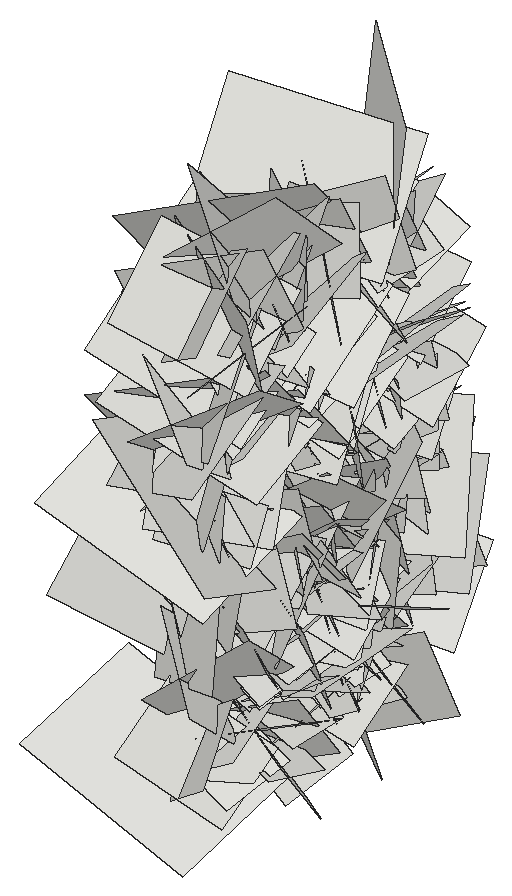
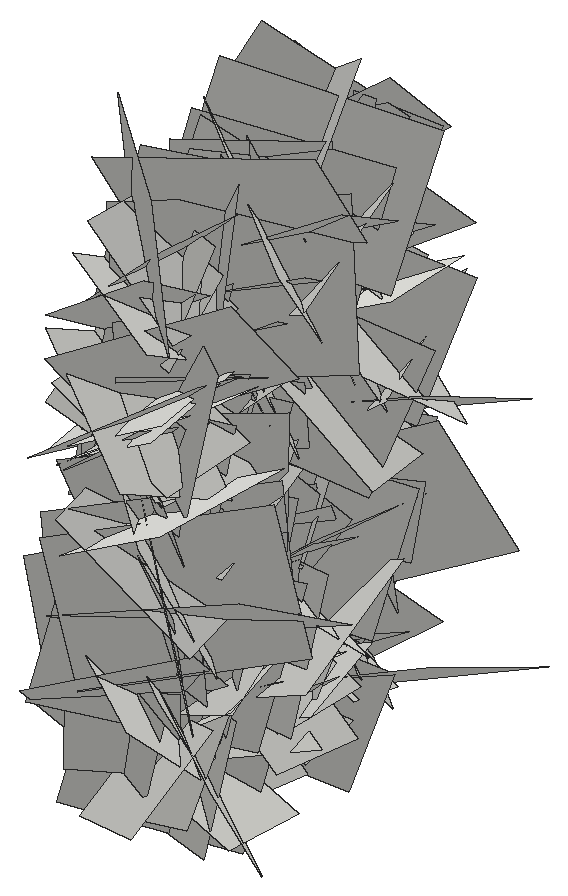
# SketchUp Ruby script. Lengths in inches.
U = 1.inch
M = Sketchup.active_model
def pt(a) = Geom::Point3d.new(a.map { |v| v * U })
def face(e, loops, mat)
  f = e.add_face(loops[0].map { |a| pt(a) })
  loops[1..].each { |l| e.add_face(l.map { |a| pt(a) }).erase! }
  f.material = f.back_material = mat if mat
  f
end
# faces: each face lists its corners as indices into pts; further lists are holes
def faces(e, pts, list, mat = nil) = list.each { |f| face(e, (f[0].is_a?(Array) ? f : [f]).map { |l| l.map { |i| pts[i] } }, mat) }
# xy, xz, yz: faces in a plane at the given z, y or x. An outline is a flat list of corners, or four numbers for a rectangle; further outlines are holes
def ring(l) = l.size == 4 ? [[l[0], l[1]], [l[2], l[1]], [l[2], l[3]], [l[0], l[3]]] : l.each_slice(2).to_a
def flat(e, list, mat, &to3) = list.each { |f| face(e, (f[0].is_a?(Array) ? f : [f]).map { |l| ring(l).map { |u, v| to3.(u, v) } }, mat) }
def xy(e, z, list, mat = nil) = flat(e, list, mat) { |x, y| [x, y, z] }
def xz(e, y, list, mat = nil) = flat(e, list, mat) { |x, z| [x, y, z] }
def yz(e, x, list, mat = nil) = flat(e, list, mat) { |y, z| [x, y, z] }
def lines(e, pts, list) = list.each { |a, b| e.add_line(pt(pts[a]), pt(pts[b])) }
# prism: a flat outline (further loops are holes) pulled along v
def prism(e, loops, v, mat = nil)
  f = face(e, loops, mat); d = Geom::Vector3d.new(v.map { |x| x * U })
  f.pushpull(f.normal.samedirection?(d) ? d.length : -d.length)
end
def box(e, o, s, mat = nil) = prism(e, [[o, [o[0] + s[0], o[1], o[2]], [o[0] + s[0], o[1] + s[1], o[2]], [o[0], o[1] + s[1], o[2]]]], [0, 0, s[2]], mat)
def at(x, y, z, deg = 0) = Geom::Transformation.translation(pt([x, y, z])) * Geom::Transformation.rotation(ORIGIN, Z_AXIS, deg.degrees)
def axes(o, x, y, z) = Geom::Transformation.new([*x, 0, *y, 0, *z, 0, *pt(o).to_a, 1])
def part(name) = M.definitions.add(name)
# library, detail: a bought-in or finely detailed component or shape, given as its bounding box
def library(name, o, s) = part(name).tap { |d| box(d.entities, o, s) }
def detail(e, o, s) = box(e.add_group.entities, o, s)
def put(e, d, t, mat = nil) = e.add_instance(d, t).tap { |i| i.material = mat if mat }
def group(e, t, mat = nil) = e.add_group.tap { |g| g.transformation = t; g.material = mat if mat }.entities
root = M.entities
c1 = part("Component\#6")
p = [[0.01,0,0],[0,3.24,4.54],[4.32,3.24,4.54],[4.33,0,0]]
faces(c1.entities,p,[[0,1,2,3]])
put(root,c1,axes([404.88,161.87,9.58],[-0.35888,-0.49511,-1.17449],[-0.11741,-1.19919,0.53746],[-1.34594,0.23663,0.26628]))
put(root,c1,axes([404.88,170.67,8.29],[-0.13658,-1.14766,-0.62909],[-0.33753,-0.58565,1.13362],[-1.34561,0.26339,-0.2205]))
put(root,c1,axes([404.88,160.65,1.35],[-0.1594,-1.22011,-0.46707],[-0.28659,-0.43091,1.2127],[-1.35486,0.2347,-0.20157]))
put(root,c1,axes([404.88,161.24,11.55],[-0.08722,-1.18104,-0.51149],[-0.30261,-0.48302,1.16122],[-1.33028,0.18731,-0.23062]))
put(root,c1,axes([404.88,161.91,24.73],[-0.20116,0.87735,-0.9177],[-0.06395,-0.93308,-0.87958],[-1.34427,-0.0869,0.17917]))
put(root,c1,axes([404.88,167.61,21.95],[-0.32344,0.31012,-1.26322],[0.1451,-1.28265,-0.34796],[-1.37111,-0.2089,0.26116]))
put(root,c1,axes([404.88,171.01,11.29],[-0.23144,-0.15428,-1.27652],[0.01824,-1.29503,0.15357],[-1.36284,0.00887,0.21884]))
put(root,c1,axes([404.88,161.07,7.88],[-0.0926,0.91308,0.78861],[-0.24837,0.76278,-0.90913],[-1.25453,-0.21841,0.12178]))
put(root,c1,axes([404.88,170.58,10.37],[-0.24309,-1.14649,0.14454],[-0.04952,0.15643,1.16674],[-1.2239,0.22139,-0.07591]))
put(root,c1,axes([404.88,165.1,2.71],[0.06092,-1.21711,0.58199],[-0.18306,0.57109,1.21136],[-1.41828,-0.12599,-0.13136]))
put(root,c1,axes([404.88,162.31,11.53],[-0.17206,0.75955,-0.87532],[-0.12131,-0.89005,-0.75111],[-1.22246,-0.01858,0.19774]))
put(root,c1,axes([404.88,157.93,15.34],[-0.27083,1.19165,0.15594],[0.0802,0.17506,-1.21378],[-1.27139,-0.2428,-0.10978]))
put(root,c1,axes([404.88,168.375,23.9],[0.0952,-0.72561,-1.04974],[-0.29336,-1.03837,0.69407],[-1.32049,0.17837,-0.22987]))
put(root,c1,axes([404.88,159.14,18.38],[-0.07521,0.79304,-0.86536],[-0.12573,-0.86735,-0.78513],[-1.23784,0.03991,0.13233]))
put(root,c1,axes([404.88,155.03,14.95],[0.10989,1.07322,0.82249],[-0.07177,0.82799,-1.07186],[-1.43147,0.04087,0.11688]))
put(root,c1,axes([404.88,166.4,18.65],[0.092,-1.19571,-0.63762],[-0.0325,-0.6405,1.19693],[-1.43603,-0.06211,-0.06794]))
put(root,c1,axes([404.88,159.69,18.96],[-0.02704,0.74145,1.09535],[0.09362,1.09406,-0.73853],[-1.39894,0.05888,-0.07059]))
put(root,c1,axes([404.88,163.36,23.49],[-0.04873,0.57368,-1.00395],[-0.12423,-1.00188,-0.56714],[-1.21936,0.07915,0.09791]))
put(root,c1,axes([404.88,162.85,15.75],[-0.04254,-1.00522,0.67204],[-0.02385,0.67292,1.00519],[-1.28151,0.02084,-0.04102]))
put(root,c1,axes([404.88,163.86,1.73],[-0.03729,0.66749,1.03354],[0.00972,1.03407,-0.66752],[-1.30413,-0.01138,-0.03452]))
put(root,c1,axes([404.88,161.03,16.77],[0.02327,0.73455,-0.90907],[-0.17416,-0.89826,-0.72978],[-1.22657,0.14148,0.08637]))
put(root,c1,axes([404.88,162.03,18.62],[-0.15865,-0.78055,-0.79386],[0.03617,-0.80384,0.78393],[-1.17956,0.08034,0.13081]))
put(root,c1,axes([404.88,161.02,12.77],[-0.04866,0.36936,-1.04237],[-0.12613,-1.03886,-0.36288],[-1.16543,0.09701,0.0828]))
put(root,c1,axes([404.88,163.21,2.24],[0.08398,-0.53221,1.10764],[-0.11648,1.10243,0.53756],[-1.29738,-0.13342,0.02343]))
put(root,c1,axes([404.88,155.93,16.01],[-0.06166,0.77521,1.08886],[0.24821,1.07895,-0.75564],[-1.39492,0.15772,-0.18259]))
put(root,c1,axes([400.91,164.09,3.1],[-0.16189,-0.51758,0.36968],[-0.06161,0.38995,0.52196],[0.67139,-0.08902,0.13704]))
put(root,c1,axes([404.88,165.97,13.03],[-0.11695,-0.23373,1.15092],[0.10796,1.14973,0.24325],[-1.24018,0.12213,-0.08736]))
put(root,c1,axes([404.88,170.79,17.67],[-0.07972,-0.69903,-0.88266],[0.01234,-0.88506,0.69994],[-1.19343,0.03754,0.0662]))
put(root,c1,axes([404.88,164.53,2.65],[-0.11418,0.95876,0.15487],[-0.16789,0.13639,-0.95453],[-1.01568,-0.13033,0.14037]))
put(root,c1,axes([404.88,165.6875,8.33],[-0.14254,-0.77018,0.64298],[-0.05856,0.65343,0.77114],[-1.06187,0.06735,-0.12884]))
put(root,c1,axes([400.91,159.77,13.93],[-0.14822,0.47929,0.38572],[0.01533,0.39801,-0.48932],[0.65196,0.0996,0.0992]))
put(root,c1,axes([404.88,164.18,5.53],[-0.00871,-1.21515,-0.1589],[0.11926,-0.15898,1.20995],[-1.29354,-0.00648,0.11262]))
put(root,c1,axes([404.88,168.99,0.33],[-0.20008,-0.71049,0.66963],[0.07161,0.67089,0.73087],[-1.03242,0.18422,-0.07908]))
put(root,c1,axes([404.88,166.625,12.7],[-0.17127,1.04033,-0.10676],[0.13463,-0.08771,-1.04688],[-1.10034,-0.17266,-0.11147]))
put(root,c1,axes([404.88,160.14,4.78],[-0.03826,-0.47304,0.81506],[-0.18962,0.80427,0.45886],[-0.98077,-0.13704,-0.12051]))
put(root,c1,axes([400.91,170.02,6.34],[-0.13634,-0.30577,-0.6303],[-0.02329,-0.63876,0.31436],[0.74222,-0.07621,-0.10592]))
put(root,c1,axes([404.88,156.14,6.5],[-0.17845,0.35117,0.84391],[-0.01887,0.85668,-0.36003],[-0.96872,-0.08137,-0.14844]))
put(root,c1,axes([404.88,163.93,5.47],[-0.11462,-1.01834,-0.26907],[0.10191,-0.2789,1.0169],[-1.11183,0.07941,0.12095]))
put(root,c1,axes([400.91,162.91,7.6875],[-0.03517,0.6334,0.29771],[-0.1292,0.28826,-0.62688],[0.73053,0.08147,-0.09654]))
put(root,c1,axes([404.88,160.62,5.12],[-0.08568,1.04485,0.18773],[0.09569,0.19436,-1.04286],[-1.1212,-0.06325,-0.10335]))
put(root,c1,axes([404.88,162.44,14.8125],[0.22172,-1.13603,-0.19278],[-0.19013,-0.22565,1.13507],[-1.20652,-0.17321,-0.21429]))
put(root,c1,axes([404.88,159.91,9.22],[0.2022,-1.20502,0.50539],[0.1049,0.52261,1.20871],[-1.38114,-0.13672,0.1658]))
put(root,c1,axes([404.88,163.57,3.71],[-0.11292,-0.2033,0.99476],[0.09749,0.99417,0.21302],[-1.07181,0.11185,-0.08542]))
put(root,c1,axes([404.88,166.01,11.8],[-0.21466,0.53877,-0.68228],[0.03009,-0.69607,-0.55809],[-0.92102,-0.14831,0.14079]))
put(root,c1,axes([404.88,168.87,14.79],[-0.03205,0.06087,-1.12787],[0.16204,-1.11767,-0.06442],[-1.18627,-0.15431,0.02167]))
put(root,c1,axes([404.88,167.18,1.59],[0.07507,-1.0991,0.32301],[0.05871,0.32653,1.09895],[-1.2129,-0.05222,0.07319]))
put(root,c1,axes([404.88,157.18,19.73],[0.07599,0.81527,0.8297],[0.084,0.82592,-0.8184],[-1.23014,0.10676,-0.00463]))
put(root,c1,axes([404.88,167.28,17.92],[0.19972,-0.96368,-0.57877],[-0.14667,-0.60226,0.95775],[-1.18251,-0.08806,-0.21655]))
put(root,c1,axes([404.88,167.22,15.375],[0.0235,-0.92066,-0.53568],[0.01768,-0.53543,0.92093],[-1.12894,-0.02755,0.00327]))
put(root,c1,axes([400.91,162.79,15.86],[-0.07285,0.46729,0.4905],[0.02436,0.49435,-0.46773],[0.71769,0.03066,0.06566]))
put(root,c1,axes([400.91,161.25,17.66],[-0.25985,0.898,-0.37026],[-0.14737,-0.41038,-0.90325],[1.01902,0.16964,-0.22504]))
put(root,c1,axes([400.91,165.96,10.85],[-0.09912,0.20412,-0.70693],[-0.02587,-0.71308,-0.20267],[0.77953,0.00229,-0.09661]))
put(root,c1,axes([404.88,169.19,10.7],[0.0913,0.46499,-1.24639],[0.29576,-1.22753,-0.43867],[-1.37875,-0.23253,-0.17663]))
put(root,c1,axes([404.88,168.14,0.12],[0.06773,-0.63363,0.78179],[-0.11595,0.77435,0.63654],[-1.06038,-0.12515,-0.01967]))
put(root,c1,axes([404.88,166.18,19.56],[0.12535,0.0531,1.28965],[0.2192,1.27754,-0.07157],[-1.35051,0.21229,0.10808]))
put(root,c1,axes([404.88,167.01,8.33],[-0.18631,0.3359,0.73427],[-0.04897,0.74605,-0.35235],[-0.8545,-0.11599,-0.1399]))
put(root,c1,axes([400.91,159.82,10.86],[-0.164,0.05549,-0.7166],[0.119,-0.72215,-0.08015],[0.75252,0.12629,-0.14349]))
put(root,c1,axes([404.88,164.72,6.23],[0.02586,0.29335,1.1723],[0.23754,1.1511,-0.29271],[-1.25874,0.22326,-0.03115]))
put(root,c1,axes([400.91,164.71,11.17],[-0.09162,-0.23701,0.75882],[-0.09076,0.76162,0.22813],[0.83777,0.05659,0.1077]))
put(root,c1,axes([400.91,167.39,12.19],[-0.06725,0.11282,-0.6237],[0.12717,-0.61335,-0.12315],[0.65971,0.12973,-0.03984]))
put(root,c1,axes([400.91,158.25,7.85],[0.01053,0.60228,-0.51533],[-0.19634,-0.49934,-0.58716],[0.81696,-0.12777,-0.13447]))
put(root,c1,axes([404.88,165.51,17.74],[-0.00528,-0.97827,-0.44464],[0.11526,-0.44282,0.97306],[-1.13321,-0.04048,0.10104]))
put(root,c1,axes([404.88,165.75,-1.09],[0.03685,-0.4153,0.96157],[0.02645,0.96216,0.41465],[-1.10996,0.00914,0.04181]))
put(root,c1,axes([404.88,167.74,3.51],[0.11337,-0.86322,0.3774],[-0.28126,0.33685,0.84566],[-0.95821,-0.201,-0.20357]))
put(root,c1,axes([404.88,161.03,4.22],[-0.00206,0.54706,-0.73945],[-0.10036,-0.73565,-0.544],[-0.96983,0.07497,0.05787]))
put(root,c1,axes([404.88,158.84,13.7],[-0.15038,-0.75335,0.50607],[0.08727,0.49942,0.76653],[-0.95804,0.16374,-0.00961]))
put(root,c1,axes([404.88,166.72,20.27],[-0.14718,0.45385,-0.66356],[-0.05291,-0.67695,-0.45256],[-0.85051,-0.03642,0.14299]))
put(root,c1,axes([400.91,158.82,19.64],[0.09205,0.73549,-0.019],[-0.17536,0.00088,-0.72213],[0.75991,-0.08889,-0.16434]))
put(root,c1,axes([404.88,169.09,13.37],[-0.12805,-0.81492,0.2825],[0.01832,0.28292,0.8235],[-0.91406,0.11983,-0.02307]))
put(root,c1,axes([400.91,159.61,12.59],[0.0897,0.16152,-0.57424],[0.01993,-0.58042,-0.16049],[0.632,-0.00462,0.08656]))
put(root,c1,axes([400.91,160.65,18.69],[0.1336,-0.1743,0.59472],[-0.06624,0.60023,0.18916],[0.65357,0.09646,-0.1024]))
put(root,c1,axes([400.91,160.54,14.42],[-0.065,-0.29459,-0.75204],[-0.0763,-0.74921,0.29935],[0.85274,-0.0895,-0.03054]))
put(root,c1,axes([400.91,161.26,10.83],[-0.08958,0.45503,-0.59155],[0.06652,-0.58889,-0.46195],[0.78829,0.10141,-0.02824]))
put(root,c1,axes([404.88,170.16,13.55],[0.14984,-1.04824,-0.22204],[-0.00627,-0.22472,1.05715],[-1.13577,-0.13705,-0.03513]))
put(root,c1,axes([400.91,160.97,6.7],[0.04912,0.73058,0.10133],[-0.09877,0.10652,-0.72536],[0.77557,-0.03271,-0.0988]))
put(root,c1,axes([404.88,163.26,10.51],[-0.09772,0.8385,-0.3881],[0.10419,-0.37892,-0.842],[-0.97385,-0.12468,-0.05114]))
put(root,c1,axes([400.91,159.79,25.07],[-0.1328,0.69586,-0.68383],[-0.18687,-0.69425,-0.67416],[1.01714,-0.03669,-0.21313]))
put(root,c1,axes([404.88,167.39,3.05],[0.22625,-1.02118,-0.283],[-0.12014,-0.30902,1.02962],[-1.11681,-0.17363,-0.16809]))
put(root,c1,axes([400.91,159.32,12.84],[0.06752,-0.16321,-0.59207],[0.0871,-0.58763,0.17083],[0.64514,0.09641,0.0389]))
put(root,c1,axes([400.91,169.73,5.36],[0.07377,0.11031,-0.61615],[0.06228,-0.61836,-0.10407],[0.66058,0.04598,0.07863]))
put(root,c1,axes([404.88,166.22,16.78],[0.0558,0.90138,-0.08554],[-0.09664,-0.07998,-0.89882],[-0.95488,0.06076,0.08597]))
put(root,c1,axes([400.91,166.8,6.58],[-0.19077,-0.84984,-0.315],[0.00737,-0.32244,0.86593],[0.9607,-0.16629,-0.0692]))
put(root,c1,axes([404.88,159.03,23.29],[0.13252,0.38295,-0.87838],[-0.10893,-0.87536,-0.39626],[-1.00987,0.14467,-0.07253]))
put(root,c1,axes([400.91,160.57,3.12],[0.03509,0.82869,0.13415],[-0.15764,0.13792,-0.81528],[0.87577,-0.00838,-0.15213]))
put(root,c1,axes([400.91,164.04,15.7],[0.03624,-0.6234,-0.24842],[0.08,-0.24359,0.62167],[0.70683,0.05954,-0.05762]))
put(root,c1,axes([404.88,170.98,12.21],[0.31631,-0.51758,-1.19288],[0.16648,-1.20059,0.56021],[-1.36826,-0.26573,-0.20761]))
put(root,c1,axes([400.91,169.83,13.22],[0.13817,-0.64015,-0.16037],[-0.03989,-0.17041,0.64965],[0.69839,0.11692,0.06883]))
put(root,c1,axes([400.91,161.46,7.67],[0.11157,-0.00104,0.59962],[0.09459,0.60203,-0.01462],[0.62852,-0.09042,-0.10424]))
put(root,c1,axes([404.88,168.08,9.41],[0.11593,0.02752,-0.90523],[-0.14705,-0.90054,-0.04413],[-0.94866,0.14295,-0.10378]))
put(root,c1,axes([400.91,169.26,18.83],[0.02849,-0.83115,-0.05333],[-0.13283,-0.05679,0.82186],[0.87278,0.01849,0.12683]))
put(root,c1,axes([400.91,165.55,15.88],[-0.02597,-0.35934,-0.67832],[0.02345,-0.67872,0.35875],[0.81334,0.00809,-0.032]))
put(root,c1,axes([400.91,167.12,21.5],[0.0656,0.35319,-0.61189],[0.00255,-0.61434,-0.35436],[0.7489,-0.02885,0.0548]))
put(root,c1,axes([404.88,164.04,2.37],[0.08884,-0.86849,0.07962],[-0.14736,0.06566,0.86256],[-0.91264,-0.09515,-0.13152]))
put(root,c1,axes([404.88,162.54,0.74],[0.05881,-0.79857,0.25436],[-0.14334,0.24305,0.79255],[-0.87675,-0.0933,-0.11251]))
put(root,c1,axes([404.88,157.37,3.29],[-0.12325,0.67494,0.21472],[-0.06797,0.20667,-0.68436],[-0.74769,-0.13004,0.02682]))
put(root,c1,axes([404.88,166.02,4.84],[0.16866,0.71959,0.68076],[-0.0323,0.69272,-0.72511],[-1.04952,0.09433,0.13172]))
put(root,c1,axes([400.91,162.4,12.14],[0.15913,-0.1111,0.71617],[-0.10617,0.72117,0.13287],[0.76084,0.12387,-0.13124]))
put(root,c1,axes([400.91,165.06,16.01],[-0.24936,0.99659,0.4051],[-0.07669,0.39908,-1.02378],[1.13774,0.24532,0.01978]))
put(root,c1,axes([400.91,164.7,6.68],[-0.19863,-0.78204,0.62344],[-0.03401,0.63866,0.7915],[1.0596,-0.1261,0.14227]))
put(root,c1,axes([404.88,166.67,11.65],[-0.03639,0.32382,0.70516],[-0.0632,0.70266,-0.32558],[-0.82009,-0.06852,-0.0062]))
put(root,c1,axes([404.88,166.25,3.34],[-0.10377,-0.78092,-0.09398],[0.04515,-0.09983,0.78516],[-0.83253,0.09192,0.05429]))
put(root,c1,axes([404.88,167.84,10.46],[0.01526,0.23241,-0.73689],[-0.14958,-0.72384,-0.23105],[-0.80526,0.13886,0.02896]))
put(root,c1,axes([404.88,164.66,7.18],[0.03191,0.54978,-0.59147],[-0.106,-0.58478,-0.54866],[-0.84939,0.09364,0.04625]))
put(root,c1,axes([404.88,155.24,20.59],[-0.01301,0.69003,0.71111],[0.211,0.69839,-0.67424],[-1.02891,0.13449,-0.14726]))
put(root,c1,axes([404.88,167.39,19.82],[-0.12929,0.6108,0.35138],[-0.02449,0.35295,-0.62154],[-0.74654,-0.11736,-0.04046]))
put(root,c1,axes([400.91,165.07,9.38],[0.13081,0.27606,-0.70722],[-0.08788,-0.70731,-0.29057],[0.79993,-0.12284,0.08373]))
put(root,c1,axes([404.88,159.79,6],[0.13547,0.51146,0.93772],[0.15367,0.92736,-0.52557],[-1.12174,0.18881,0.04125]))
put(root,c1,axes([404.88,159.9,13.67],[0.02397,0.44215,0.82689],[0.11898,0.8199,-0.44149],[-0.98679,0.1096,-0.03314]))
put(root,c1,axes([400.91,164.44,22.83],[-0.02931,-0.02413,-0.88007],[-0.04764,-0.87932,0.02552],[0.93201,-0.0457,-0.02637]))
put(root,c1,axes([404.88,168.54,15.47],[0.051,0.16682,-0.79913],[-0.09039,-0.79511,-0.17112],[-0.86061,0.0934,-0.02938]))
put(root,c1,axes([404.88,155.625,2.89],[-0.13104,0.56412,0.5606],[0.11872,0.57403,-0.55293],[-0.83462,-0.00692,-0.16667]))
put(root,c1,axes([404.88,163.43,17.5],[0.07736,-0.30856,0.98844],[0.18729,0.98007,0.2929],[-1.08152,0.14765,0.12143]))
put(root,c1,axes([400.91,163.43,17.5],[-0.07736,-0.30856,0.98844],[-0.18729,0.98007,0.2929],[1.08152,0.14765,0.12143]))
put(root,c1,axes([400.91,155.625,2.89],[0.13104,0.56412,0.5606],[-0.11872,0.57403,-0.55293],[0.83462,-0.00692,-0.16667]))
put(root,c1,axes([400.91,168.54,15.47],[-0.051,0.16682,-0.79913],[0.09039,-0.79511,-0.17112],[0.86061,0.0934,-0.02938]))
put(root,c1,axes([404.88,164.44,22.83],[0.02931,-0.02413,-0.88007],[0.04764,-0.87932,0.02552],[-0.93201,-0.0457,-0.02637]))
put(root,c1,axes([400.91,159.9,13.67],[-0.02397,0.44215,0.82689],[-0.11898,0.8199,-0.44149],[0.98679,0.1096,-0.03314]))
put(root,c1,axes([400.91,159.79,6],[-0.13547,0.51146,0.93772],[-0.15367,0.92736,-0.52557],[1.12174,0.18881,0.04125]))
put(root,c1,axes([404.88,165.07,9.38],[-0.13081,0.27606,-0.70722],[0.08788,-0.70731,-0.29057],[-0.79993,-0.12284,0.08373]))
put(root,c1,axes([400.91,167.39,19.82],[0.12929,0.6108,0.35138],[0.02449,0.35295,-0.62154],[0.74654,-0.11736,-0.04046]))
put(root,c1,axes([400.91,155.24,20.59],[0.01301,0.69003,0.71111],[-0.211,0.69839,-0.67424],[1.02891,0.13449,-0.14726]))
put(root,c1,axes([400.91,164.66,7.18],[-0.03191,0.54978,-0.59147],[0.106,-0.58478,-0.54866],[0.84939,0.09364,0.04625]))
put(root,c1,axes([400.91,167.84,10.46],[-0.01526,0.23241,-0.73689],[0.14958,-0.72384,-0.23105],[0.80526,0.13886,0.02896]))
put(root,c1,axes([400.91,166.25,3.34],[0.10377,-0.78092,-0.09398],[-0.04515,-0.09983,0.78516],[0.83253,0.09192,0.05429]))
put(root,c1,axes([400.91,166.67,11.65],[0.03639,0.32382,0.70516],[0.0632,0.70266,-0.32558],[0.82009,-0.06852,-0.0062]))
put(root,c1,axes([404.88,164.7,6.68],[0.19863,-0.78204,0.62344],[0.03401,0.63866,0.7915],[-1.0596,-0.1261,0.14227]))
put(root,c1,axes([404.88,165.06,16.01],[0.24936,0.99659,0.4051],[0.07669,0.39908,-1.02378],[-1.13774,0.24532,0.01978]))
put(root,c1,axes([404.88,162.4,12.14],[-0.15913,-0.1111,0.71617],[0.10617,0.72117,0.13287],[-0.76084,0.12387,-0.13124]))
put(root,c1,axes([400.91,166.02,4.84],[-0.16866,0.71959,0.68076],[0.0323,0.69272,-0.72511],[1.04952,0.09433,0.13172]))
put(root,c1,axes([400.91,157.37,3.29],[0.12325,0.67494,0.21472],[0.06797,0.20667,-0.68436],[0.74769,-0.13004,0.02682]))
put(root,c1,axes([400.91,162.54,0.74],[-0.05881,-0.79857,0.25436],[0.14334,0.24305,0.79255],[0.87675,-0.0933,-0.11251]))
put(root,c1,axes([400.91,164.04,2.37],[-0.08884,-0.86849,0.07962],[0.14736,0.06566,0.86256],[0.91264,-0.09515,-0.13152]))
put(root,c1,axes([404.88,167.12,21.5],[-0.0656,0.35319,-0.61189],[-0.00255,-0.61434,-0.35436],[-0.7489,-0.02885,0.0548]))
put(root,c1,axes([404.88,165.55,15.88],[0.02597,-0.35934,-0.67832],[-0.02345,-0.67872,0.35875],[-0.81334,0.00809,-0.032]))
put(root,c1,axes([404.88,169.26,18.83],[-0.02849,-0.83115,-0.05333],[0.13283,-0.05679,0.82186],[-0.87278,0.01849,0.12683]))
put(root,c1,axes([400.91,168.08,9.41],[-0.11593,0.02752,-0.90523],[0.14705,-0.90054,-0.04413],[0.94866,0.14295,-0.10378]))
put(root,c1,axes([404.88,161.46,7.67],[-0.11157,-0.00104,0.59962],[-0.09459,0.60203,-0.01462],[-0.62852,-0.09042,-0.10424]))
put(root,c1,axes([404.88,169.83,13.22],[-0.13817,-0.64015,-0.16037],[0.03989,-0.17041,0.64965],[-0.69839,0.11692,0.06883]))
put(root,c1,axes([400.91,170.98,12.21],[-0.31631,-0.51758,-1.19288],[-0.16648,-1.20059,0.56021],[1.36826,-0.26573,-0.20761]))
put(root,c1,axes([404.88,164.04,15.7],[-0.03624,-0.6234,-0.24842],[-0.08,-0.24359,0.62167],[-0.70683,0.05954,-0.05762]))
put(root,c1,axes([404.88,160.57,3.12],[-0.03509,0.82869,0.13415],[0.15764,0.13792,-0.81528],[-0.87577,-0.00838,-0.15213]))
put(root,c1,axes([400.91,159.03,23.29],[-0.13252,0.38295,-0.87838],[0.10893,-0.87536,-0.39626],[1.00987,0.14467,-0.07253]))
put(root,c1,axes([404.88,166.8,6.58],[0.19077,-0.84984,-0.315],[-0.00737,-0.32244,0.86593],[-0.9607,-0.16629,-0.0692]))
put(root,c1,axes([400.91,166.22,16.78],[-0.0558,0.90138,-0.08554],[0.09664,-0.07998,-0.89882],[0.95488,0.06076,0.08597]))
put(root,c1,axes([404.88,169.73,5.36],[-0.07377,0.11031,-0.61615],[-0.06228,-0.61836,-0.10407],[-0.66058,0.04598,0.07863]))
put(root,c1,axes([404.88,159.32,12.84],[-0.06752,-0.16321,-0.59207],[-0.0871,-0.58763,0.17083],[-0.64514,0.09641,0.0389]))
put(root,c1,axes([400.91,167.39,3.05],[-0.22625,-1.02118,-0.283],[0.12014,-0.30902,1.02962],[1.11681,-0.17363,-0.16809]))
put(root,c1,axes([404.88,159.79,25.07],[0.1328,0.69586,-0.68383],[0.18687,-0.69425,-0.67416],[-1.01714,-0.03669,-0.21313]))
put(root,c1,axes([400.91,163.26,10.51],[0.09772,0.8385,-0.3881],[-0.10419,-0.37892,-0.842],[0.97385,-0.12468,-0.05114]))
put(root,c1,axes([404.88,160.97,6.7],[-0.04912,0.73058,0.10133],[0.09877,0.10652,-0.72536],[-0.77557,-0.03271,-0.0988]))
put(root,c1,axes([400.91,170.16,13.55],[-0.14984,-1.04824,-0.22204],[0.00627,-0.22472,1.05715],[1.13577,-0.13705,-0.03513]))
put(root,c1,axes([404.88,161.26,10.83],[0.08958,0.45503,-0.59155],[-0.06652,-0.58889,-0.46195],[-0.78829,0.10141,-0.02824]))
put(root,c1,axes([404.88,160.54,14.42],[0.065,-0.29459,-0.75204],[0.0763,-0.74921,0.29935],[-0.85274,-0.0895,-0.03054]))
put(root,c1,axes([404.88,160.65,18.69],[-0.1336,-0.1743,0.59472],[0.06624,0.60023,0.18916],[-0.65357,0.09646,-0.1024]))
put(root,c1,axes([404.88,159.61,12.59],[-0.0897,0.16152,-0.57424],[-0.01993,-0.58042,-0.16049],[-0.632,-0.00462,0.08656]))
put(root,c1,axes([400.91,169.09,13.37],[0.12805,-0.81492,0.2825],[-0.01832,0.28292,0.8235],[0.91406,0.11983,-0.02307]))
put(root,c1,axes([404.88,158.82,19.64],[-0.09205,0.73549,-0.019],[0.17536,0.00088,-0.72213],[-0.75991,-0.08889,-0.16434]))
put(root,c1,axes([400.91,166.72,20.27],[0.14718,0.45385,-0.66356],[0.05291,-0.67695,-0.45256],[0.85051,-0.03642,0.14299]))
put(root,c1,axes([400.91,158.84,13.7],[0.15038,-0.75335,0.50607],[-0.08727,0.49942,0.76653],[0.95804,0.16374,-0.00961]))
put(root,c1,axes([400.91,161.03,4.22],[0.00206,0.54706,-0.73945],[0.10036,-0.73565,-0.544],[0.96983,0.07497,0.05787]))
put(root,c1,axes([400.91,167.74,3.51],[-0.11337,-0.86322,0.3774],[0.28126,0.33685,0.84566],[0.95821,-0.201,-0.20357]))
put(root,c1,axes([400.91,165.75,-1.09],[-0.03685,-0.4153,0.96157],[-0.02645,0.96216,0.41465],[1.10996,0.00914,0.04181]))
put(root,c1,axes([400.91,165.51,17.74],[0.00528,-0.97827,-0.44464],[-0.11526,-0.44282,0.97306],[1.13321,-0.04048,0.10104]))
put(root,c1,axes([404.88,158.25,7.85],[-0.01053,0.60228,-0.51533],[0.19634,-0.49934,-0.58716],[-0.81696,-0.12777,-0.13447]))
put(root,c1,axes([404.88,167.39,12.19],[0.06725,0.11282,-0.6237],[-0.12717,-0.61335,-0.12315],[-0.65971,0.12973,-0.03984]))
put(root,c1,axes([404.88,164.71,11.17],[0.09162,-0.23701,0.75882],[0.09076,0.76162,0.22813],[-0.83777,0.05659,0.1077]))
put(root,c1,axes([400.91,164.72,6.23],[-0.02586,0.29335,1.1723],[-0.23754,1.1511,-0.29271],[1.25874,0.22326,-0.03115]))
put(root,c1,axes([404.88,159.82,10.86],[0.164,0.05549,-0.7166],[-0.119,-0.72215,-0.08015],[-0.75252,0.12629,-0.14349]))
